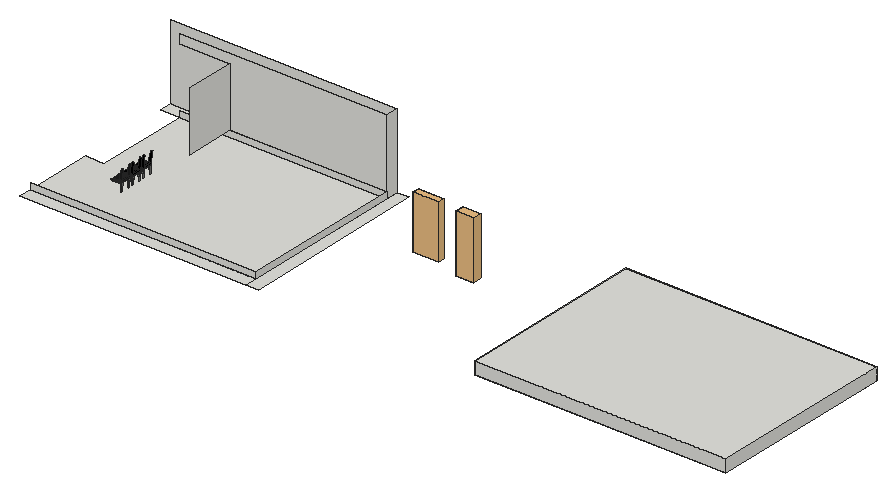
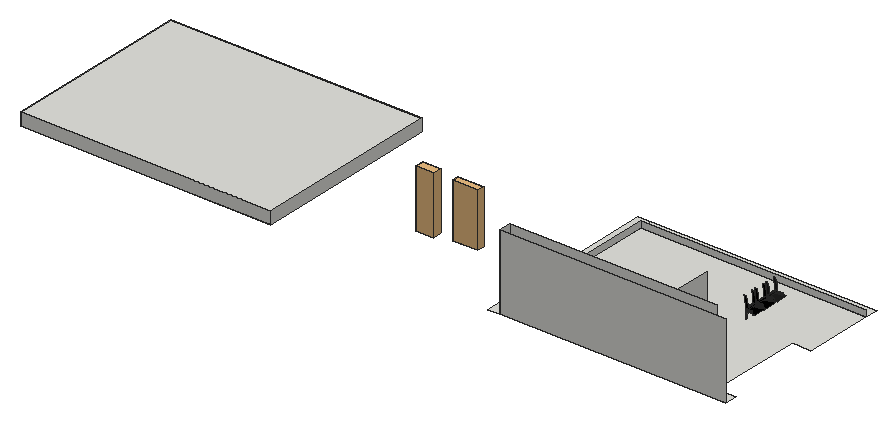
# SketchUp Ruby script. Lengths in inches.
U = 1.inch
M = Sketchup.active_model
def pt(a) = Geom::Point3d.new(a.map { |v| v * U })
def face(e, loops, mat)
  f = e.add_face(loops[0].map { |a| pt(a) })
  loops[1..].each { |l| e.add_face(l.map { |a| pt(a) }).erase! }
  f.material = f.back_material = mat if mat
  f
end
# faces: each face lists its corners as indices into pts; further lists are holes
def faces(e, pts, list, mat = nil) = list.each { |f| face(e, (f[0].is_a?(Array) ? f : [f]).map { |l| l.map { |i| pts[i] } }, mat) }
# xy, xz, yz: faces in a plane at the given z, y or x. An outline is a flat list of corners, or four numbers for a rectangle; further outlines are holes
def ring(l) = l.size == 4 ? [[l[0], l[1]], [l[2], l[1]], [l[2], l[3]], [l[0], l[3]]] : l.each_slice(2).to_a
def flat(e, list, mat, &to3) = list.each { |f| face(e, (f[0].is_a?(Array) ? f : [f]).map { |l| ring(l).map { |u, v| to3.(u, v) } }, mat) }
def xy(e, z, list, mat = nil) = flat(e, list, mat) { |x, y| [x, y, z] }
def xz(e, y, list, mat = nil) = flat(e, list, mat) { |x, z| [x, y, z] }
def yz(e, x, list, mat = nil) = flat(e, list, mat) { |y, z| [x, y, z] }
def lines(e, pts, list) = list.each { |a, b| e.add_line(pt(pts[a]), pt(pts[b])) }
# prism: a flat outline (further loops are holes) pulled along v
def prism(e, loops, v, mat = nil)
  f = face(e, loops, mat); d = Geom::Vector3d.new(v.map { |x| x * U })
  f.pushpull(f.normal.samedirection?(d) ? d.length : -d.length)
end
def box(e, o, s, mat = nil) = prism(e, [[o, [o[0] + s[0], o[1], o[2]], [o[0] + s[0], o[1] + s[1], o[2]], [o[0], o[1] + s[1], o[2]]]], [0, 0, s[2]], mat)
def at(x, y, z, deg = 0) = Geom::Transformation.translation(pt([x, y, z])) * Geom::Transformation.rotation(ORIGIN, Z_AXIS, deg.degrees)
def axes(o, x, y, z) = Geom::Transformation.new([*x, 0, *y, 0, *z, 0, *pt(o).to_a, 1])
def part(name) = M.definitions.add(name)
# library, detail: a bought-in or finely detailed component or shape, given as its bounding box
def library(name, o, s) = part(name).tap { |d| box(d.entities, o, s) }
def detail(e, o, s) = box(e.add_group.entities, o, s)
def put(e, d, t, mat = nil) = e.add_instance(d, t).tap { |i| i.material = mat if mat }
def group(e, t, mat = nil) = e.add_group.tap { |g| g.transformation = t; g.material = mat if mat }.entities
root = M.entities
M.materials.add("Color_008").color = [30, 30, 30]
M.materials.add("[Color M08]").color = [30, 30, 30]
M.materials.add("[Color M09]").color = [0, 0, 0]
M.materials.add("[Metal Seamed]").color = [118, 119, 115]
c1 = library("Group\#2",[0,0,0],[48.53,12.58,103.73])
c2 = library("Group\#1",[0,0,0],[34.5,17.48,110.79])
box(root,[894.9375,0,0],[480,360,24])
xy(root,0,[[24,0,456,24],[456,0,480,360],[24,24,24,156,60,156,60,336,456,336,456,24],[24,336,456,360]])
xy(root,12,[[146.137,88.857,146.954,89.674],[146.137,105.091,146.954,105.908],[146.137,114.763,146.954,115.58],[146.137,130.997,146.954,131.814],[146.137,140.669,146.954,141.485],
  [146.137,156.903,146.954,157.72]],"Color_008")
xy(root,26.704,[[145.473,88.193,147.618,90.338],[145.473,104.427,147.618,106.572],[145.473,114.098,147.618,116.244],[145.473,130.333,147.618,132.478],[145.473,140.004,147.618,142.15],
  [145.473,156.239,147.618,158.384]],"Color_008")
xy(root,26.704,[[132.315,87.045,130.608,87.058,128.902,87.101,127.197,87.171,129.342,87.171,129.342,89.317,127.197,89.317,127.197,105.448,129.342,105.448,129.342,107.593,127.197,107.593,128.902,107.664,130.608,107.706,132.315,107.72,134.022,107.706,135.728,107.663,137.433,107.592,139.137,107.493,140.839,107.365,142.538,107.209,144.235,107.025,145.929,106.8125,147.618,106.572,145.473,106.572,145.473,104.427,147.618,104.427,147.618,90.338,145.473,90.338,145.473,88.193,147.618,88.193,145.929,87.952,144.235,87.74,142.538,87.556,140.839,87.4,139.137,87.272,137.433,87.173,135.728,87.102,134.022,87.059]],"[Color M08]")
xy(root,26.704,[[132.315,112.95,130.608,112.964,128.902,113.007,127.197,113.077,129.342,113.077,129.342,115.223,127.197,115.223,127.197,131.354,129.342,131.354,129.342,133.499,127.197,133.499,128.902,133.57,130.608,133.612,132.315,133.626,134.022,133.612,135.728,133.569,137.433,133.498,139.137,133.398,140.839,133.271,142.538,133.115,144.235,132.931,145.929,132.718,147.618,132.478,145.473,132.478,145.473,130.333,147.618,130.333,147.618,116.244,145.473,116.244,145.473,114.098,147.618,114.098,145.929,113.858,144.235,113.646,142.538,113.462,140.839,113.306,139.137,113.178,137.433,113.079,135.728,113.008,134.022,112.965],[132.315,138.856,130.608,138.87,128.902,138.913,127.197,138.983,129.342,138.983,129.342,141.129,127.197,141.129,127.197,157.26,129.342,157.26,129.342,159.405,127.197,159.405,128.902,159.476,130.608,159.518,132.315,159.532,134.022,159.517,135.728,159.475,137.433,159.404,139.137,159.304,140.839,159.177,142.538,159.021,144.235,158.837,145.929,158.624,147.618,158.384,145.473,158.384,145.473,156.239,147.618,156.239,147.618,142.15,145.473,142.15,145.473,140.004,147.618,140.004,145.929,139.764,144.235,139.552,142.538,139.367,140.839,139.212,139.137,139.084,137.433,138.984,135.728,138.913,134.022,138.871]],"[Color M09]")
xy(root,28.845,[[144.082,88.193,147.618,106.572]],"[Color M08]")
xy(root,28.845,[[144.082,114.098,147.618,132.478],[144.082,140.004,147.618,158.384]],"[Color M09]")
xz(root,24,[[24,0,456,12]])
xz(root,88.193,[[144.082,28.845,143.95,30.816,143.898,32.79,143.926,34.764,144.034,36.736,144.222,38.701,144.488,40.658,144.834,42.602,145.258,44.53,145.759,46.44,146.337,48.328,146.991,50.191,147.719,52.027,150.17,52.027,149.772,50.121,149.407,48.208,149.076,46.29,148.779,44.365,148.515,42.436,148.285,40.503,148.089,38.566,147.927,36.626,147.799,34.683,147.705,32.738,147.645,30.792,147.618,28.845]],"[Color M08]")
xz(root,106.572,[[144.082,28.845,147.618,28.845,147.645,30.792,147.705,32.738,147.799,34.683,147.927,36.626,148.089,38.566,148.285,40.503,148.515,42.436,148.779,44.365,149.076,46.29,149.407,48.208,149.772,50.121,150.17,52.027,147.719,52.027,146.991,50.191,146.337,48.328,145.759,46.44,145.258,44.53,144.834,42.602,144.488,40.658,144.222,38.701,144.034,36.736,143.926,34.764,143.898,32.79,143.95,30.816]],"[Color M08]")
xz(root,114.098,[[144.082,28.845,143.95,30.816,143.898,32.79,143.926,34.764,144.034,36.736,144.222,38.701,144.488,40.658,144.834,42.602,145.258,44.53,145.759,46.44,146.337,48.328,146.991,50.191,147.719,52.027,150.17,52.027,149.772,50.121,149.407,48.208,149.076,46.29,148.779,44.365,148.515,42.436,148.285,40.503,148.089,38.566,147.927,36.626,147.799,34.683,147.705,32.738,147.645,30.792,147.618,28.845]],"[Color M09]")
xz(root,132.478,[[144.082,28.845,147.618,28.845,147.645,30.792,147.705,32.738,147.799,34.683,147.927,36.626,148.089,38.566,148.285,40.503,148.515,42.436,148.779,44.365,149.076,46.29,149.407,48.208,149.772,50.121,150.17,52.027,147.719,52.027,146.991,50.191,146.337,48.328,145.759,46.44,145.258,44.53,144.834,42.602,144.488,40.658,144.222,38.701,144.034,36.736,143.926,34.764,143.898,32.79,143.95,30.816]],"[Color M09]")
xz(root,140.004,[[144.082,28.845,143.95,30.816,143.898,32.79,143.926,34.764,144.034,36.736,144.222,38.701,144.488,40.658,144.834,42.602,145.258,44.53,145.759,46.44,146.337,48.328,146.991,50.191,147.719,52.027,150.17,52.027,149.772,50.121,149.407,48.208,149.076,46.29,148.779,44.365,148.515,42.436,148.285,40.503,148.089,38.566,147.927,36.626,147.799,34.683,147.705,32.738,147.645,30.792,147.618,28.845]],"[Color M09]")
xz(root,158.384,[[144.082,28.845,147.618,28.845,147.645,30.792,147.705,32.738,147.799,34.683,147.927,36.626,148.089,38.566,148.285,40.503,148.515,42.436,148.779,44.365,149.076,46.29,149.407,48.208,149.772,50.121,150.17,52.027,147.719,52.027,146.991,50.191,146.337,48.328,145.759,46.44,145.258,44.53,144.834,42.602,144.488,40.658,144.222,38.701,144.034,36.736,143.926,34.764,143.898,32.79,143.95,30.816]],"[Color M09]")
xz(root,336,[[60,0,456,12],[156,12,456,12,456,144,60,144,60,126,156,126]])
xz(root,360,[[24,0,456,144]])
yz(root,147.618,[[88.193,26.704,106.572,28.845]],"[Color M08]")
yz(root,147.618,[[114.098,26.704,132.478,28.845],[140.004,26.704,158.384,28.845]],"[Color M09]")
yz(root,156,[[240,12,336,126]])
yz(root,456,[[24,0,336,12],[336,0,360,144]])
p = [[145.473,90.338,26.704],[146.137,89.674,12],[146.137,88.857,12],[145.473,88.193,26.704],[146.954,88.857,12],[147.618,88.193,26.704],
  [146.954,89.674,12],[147.618,90.338,26.704],[146.137,105.091,12],[145.473,104.427,26.704],[145.473,106.572,26.704],[146.137,105.908,12],
  [146.954,105.091,12],[147.618,104.427,26.704],[146.954,105.908,12],[147.618,106.572,26.704],[145.473,116.244,26.704],[146.137,115.58,12],
  [146.137,114.763,12],[145.473,114.098,26.704],[146.954,114.763,12],[147.618,114.098,26.704],[146.954,115.58,12],[147.618,116.244,26.704],
  [146.137,130.997,12],[145.473,130.333,26.704],[145.473,132.478,26.704],[146.137,131.814,12],[146.954,130.997,12],[147.618,130.333,26.704],
  [146.954,131.814,12],[147.618,132.478,26.704],[145.473,142.15,26.704],[146.137,141.485,12],[146.137,140.669,12],[145.473,140.004,26.704],
  [146.954,140.669,12],[147.618,140.004,26.704],[146.954,141.485,12],[147.618,142.15,26.704],[146.137,156.903,12],[145.473,156.239,26.704],
  [145.473,158.384,26.704],[146.137,157.72,12],[146.954,156.903,12],[147.618,156.239,26.704],[146.954,157.72,12],[147.618,158.384,26.704],
  [135.728,87.102,28.845],[135.728,87.102,26.704],[134.022,87.059,26.704],[134.022,87.059,28.845],[137.433,87.173,26.704],[137.433,87.173,28.845],
  [139.137,87.272,26.704],[139.137,87.272,28.845],[140.839,87.4,26.704],[140.839,87.4,28.845],[142.538,87.556,26.704],[142.538,87.556,28.845],
  [144.235,87.74,26.704],[144.235,87.74,28.845],[145.929,87.952,26.704],[145.929,87.952,28.845],[147.618,88.193,28.845],[145.929,106.8125,26.704],
  [145.929,106.8125,28.845],[147.618,106.572,28.845],[144.235,107.025,26.704],[144.235,107.025,28.845],[142.538,107.209,26.704],[142.538,107.209,28.845],
  [140.839,107.365,26.704],[140.839,107.365,28.845],[139.137,107.493,26.704],[139.137,107.493,28.845],[137.433,107.592,26.704],[137.433,107.592,28.845],
  [135.728,107.663,26.704],[135.728,107.663,28.845],[134.022,107.706,28.845],[134.022,107.706,26.704],[135.728,113.008,28.845],[135.728,113.008,26.704],
  [134.022,112.965,26.704],[134.022,112.965,28.845],[137.433,113.079,26.704],[137.433,113.079,28.845],[139.137,113.178,26.704],[139.137,113.178,28.845],
  [140.839,113.306,26.704],[140.839,113.306,28.845],[142.538,113.462,26.704],[142.538,113.462,28.845],[144.235,113.646,26.704],[144.235,113.646,28.845],
  [145.929,113.858,26.704],[145.929,113.858,28.845],[147.618,114.098,28.845],[145.929,132.718,26.704],[145.929,132.718,28.845],[147.618,132.478,28.845],
  [144.235,132.931,26.704],[144.235,132.931,28.845],[142.538,133.115,26.704],[142.538,133.115,28.845],[140.839,133.271,26.704],[140.839,133.271,28.845],
  [139.137,133.398,26.704],[139.137,133.398,28.845],[137.433,133.498,26.704],[137.433,133.498,28.845],[135.728,133.569,26.704],[135.728,133.569,28.845],
  [134.022,133.612,28.845],[134.022,133.612,26.704],[135.728,138.913,28.845],[135.728,138.913,26.704],[134.022,138.871,26.704],[134.022,138.871,28.845],
  [137.433,138.984,26.704],[137.433,138.984,28.845],[139.137,139.084,26.704],[139.137,139.084,28.845],[140.839,139.212,26.704],[140.839,139.212,28.845],
  [142.538,139.367,26.704],[142.538,139.367,28.845],[144.235,139.552,26.704],[144.235,139.552,28.845],[145.929,139.764,26.704],[145.929,139.764,28.845],
  [147.618,140.004,28.845],[145.929,158.624,26.704],[145.929,158.624,28.845],[147.618,158.384,28.845],[144.235,158.837,26.704],[144.235,158.837,28.845],
  [142.538,159.021,26.704],[142.538,159.021,28.845],[140.839,159.177,26.704],[140.839,159.177,28.845],[139.137,159.304,26.704],[139.137,159.304,28.845],
  [137.433,159.404,26.704],[137.433,159.404,28.845],[135.728,159.475,26.704],[135.728,159.475,28.845],[134.022,159.517,28.845],[134.022,159.517,26.704],
  [135.728,87.111,28.992],[134.021,87.069,28.992],[137.433,87.182,28.992],[139.136,87.282,28.992],[140.838,87.409,28.992],[142.538,87.565,28.992],
  [144.234,87.749,28.992],[145.927,87.962,28.992],[147.609,88.201,28.992],[143.95,88.193,30.816],[144.082,88.193,28.845],[144.082,106.572,28.845],
  [143.95,106.572,30.816],[147.609,106.564,28.992],[147.645,88.193,30.792],[147.645,106.572,30.792],[145.927,106.803,28.992],[144.234,107.015,28.992],
  [142.538,107.199,28.992],[140.838,107.355,28.992],[139.136,107.483,28.992],[137.433,107.582,28.992],[135.728,107.653,28.992],[134.021,107.696,28.992],
  [135.728,113.017,28.992],[134.021,112.974,28.992],[137.433,113.088,28.992],[139.136,113.1875,28.992],[140.838,113.315,28.992],[142.538,113.471,28.992],
  [144.234,113.655,28.992],[145.927,113.868,28.992],[147.609,114.107,28.992],[143.95,114.098,30.816],[144.082,114.098,28.845],[144.082,132.478,28.845],
  [143.95,132.478,30.816],[147.609,132.47,28.992],[147.645,114.098,30.792],[147.645,132.478,30.792],[145.927,132.709,28.992],[144.234,132.921,28.992],
  [142.538,133.105,28.992],[140.838,133.261,28.992],[139.136,133.389,28.992],[137.433,133.488,28.992],[135.728,133.559,28.992],[134.021,133.602,28.992],
  [135.728,138.923,28.992],[134.021,138.88,28.992],[137.433,138.994,28.992],[139.136,139.093,28.992],[140.838,139.221,28.992],[142.538,139.377,28.992],
  [144.234,139.561,28.992],[145.927,139.773,28.992],[147.609,140.013,28.992],[143.95,140.004,30.816],[144.082,140.004,28.845],[144.082,158.384,28.845],
  [143.95,158.384,30.816],[147.609,158.376,28.992],[147.645,140.004,30.792],[147.645,158.384,30.792],[145.927,158.615,28.992],[144.234,158.827,28.992],
  [142.538,159.011,28.992],[140.838,159.167,28.992],[139.136,159.295,28.992],[137.433,159.394,28.992],[135.728,159.465,28.992],[134.021,159.508,28.992],
  [135.726,87.14,29.137],[134.021,87.097,29.137],[137.431,87.211,29.137],[139.134,87.31,29.137],[140.836,87.438,29.137],[142.535,87.594,29.137],
  [144.231,87.778,29.137],[145.924,87.99,29.137],[147.58,88.226,29.137],[147.58,106.539,29.137],[147.58,97.382,29.137],[145.924,106.774,29.137],
  [144.231,106.987,29.137],[142.535,107.171,29.137],[140.836,107.327,29.137],[139.134,107.454,29.137],[137.431,107.554,29.137],[135.727,107.625,29.137],
  [134.021,107.667,29.137],[135.726,113.046,29.137],[134.021,113.003,29.137],[137.431,113.117,29.137],[139.134,113.216,29.137],[140.836,113.344,29.137],
  [142.535,113.5,29.137],[144.231,113.684,29.137],[145.924,113.896,29.137],[147.58,114.132,29.137],[147.58,132.445,29.137],[147.58,123.288,29.137],
  [145.924,132.68,29.137],[144.231,132.893,29.137],[142.535,133.077,29.137],[140.836,133.233,29.137],[139.134,133.36,29.137],[137.431,133.46,29.137],
  [135.727,133.531,29.137],[134.021,133.573,29.137],[135.726,138.952,29.137],[134.021,138.909,29.137],[137.431,139.023,29.137],[139.134,139.122,29.137],
  [140.836,139.25,29.137],[142.535,139.406,29.137],[144.231,139.59,29.137],[145.924,139.802,29.137],[147.58,140.038,29.137],[147.58,158.351,29.137],
  [147.58,149.194,29.137],[145.924,158.586,29.137],[144.231,158.798,29.137],[142.535,158.983,29.137],[140.836,159.138,29.137],[139.134,159.266,29.137],
  [137.431,159.365,29.137],[135.727,159.436,29.137],[134.021,159.479,29.137],[134.02,87.145,29.276],[135.724,87.187,29.276],[137.429,87.258,29.276],
  [135.726,87.187,29.276],[139.131,87.358,29.276],[140.832,87.485,29.276],[142.53,87.641,29.276],[144.225,87.825,29.276],[145.917,88.037,29.276],
  [147.533,88.267,29.276],[147.533,97.382,29.276],[147.533,106.498,29.276],[145.917,106.728,29.276],[144.225,106.94,29.276],[142.53,107.124,29.276],
  [140.832,107.279,29.276],[139.131,107.407,29.276],[137.429,107.506,29.276],[135.724,107.577,29.276],[135.726,107.577,29.276],[134.02,107.62,29.276],
  [134.02,113.05,29.276],[135.724,113.093,29.276],[137.429,113.164,29.276],[135.726,113.093,29.276],[139.131,113.263,29.276],[140.832,113.391,29.276],
  [142.53,113.547,29.276],[144.225,113.731,29.276],[145.917,113.943,29.276],[147.533,114.173,29.276],[147.533,123.288,29.276],[147.533,132.404,29.276],
  [145.917,132.633,29.276],[144.225,132.846,29.276],[142.53,133.03,29.276],[140.832,133.185,29.276],[139.131,133.313,29.276],[137.429,133.412,29.276],
  [135.724,133.483,29.276],[135.726,133.483,29.276],[134.02,133.526,29.276],[134.02,138.956,29.276],[135.724,138.999,29.276],[137.429,139.07,29.276],
  [135.726,138.999,29.276],[139.131,139.169,29.276],[140.832,139.297,29.276],[142.53,139.453,29.276],[144.225,139.637,29.276],[145.917,139.849,29.276],
  [147.533,140.079,29.276],[147.533,149.194,29.276],[147.533,158.31,29.276],[145.917,158.539,29.276],[144.225,158.751,29.276],[142.53,158.935,29.276],
  [140.832,159.091,29.276],[139.131,159.219,29.276],[137.429,159.318,29.276],[135.724,159.389,29.276],[135.726,159.389,29.276],[134.02,159.432,29.276],
  [134.019,87.21,29.408],[135.722,87.252,29.408],[135.724,87.252,29.408],[137.426,87.323,29.408],[139.127,87.423,29.408],[140.826,87.55,29.408],
  [142.523,87.706,29.408],[144.218,87.89,29.408],[145.909,88.102,29.408],[147.468,88.323,29.408],[147.468,97.382,29.408],[147.468,106.441,29.408],
  [145.909,106.663,29.408],[144.218,106.875,29.408],[142.523,107.059,29.408],[140.826,107.215,29.408],[139.127,107.342,29.408],[137.426,107.441,29.408],
  [135.724,107.512,29.408],[135.722,107.512,29.408],[134.019,107.555,29.408],[134.019,113.116,29.408],[135.722,113.158,29.408],[135.724,113.158,29.408],
  [137.426,113.229,29.408],[139.127,113.328,29.408],[140.826,113.456,29.408],[142.523,113.612,29.408],[144.218,113.795,29.408],[145.909,114.007,29.408],
  [147.468,114.229,29.408],[147.468,123.288,29.408],[147.468,132.347,29.408],[145.909,132.569,29.408],[144.218,132.781,29.408],[142.523,132.965,29.408],
  [140.826,133.121,29.408],[139.127,133.248,29.408],[137.426,133.347,29.408],[135.724,133.418,29.408],[135.722,133.418,29.408],[134.019,133.461,29.408],
  [134.019,139.021,29.408],[135.722,139.064,29.408],[135.724,139.064,29.408],[137.426,139.135,29.408],[139.127,139.234,29.408],[140.826,139.362,29.408],
  [142.523,139.517,29.408],[144.218,139.701,29.408],[145.909,139.913,29.408],[147.468,140.135,29.408],[147.468,149.194,29.408],[147.468,158.253,29.408],
  [145.909,158.475,29.408],[144.218,158.687,29.408],[142.523,158.871,29.408],[140.826,159.026,29.408],[139.127,159.154,29.408],[137.426,159.253,29.408],
  [135.722,159.324,29.408],[134.019,159.367,29.408],[135.724,159.324,29.408],[134.018,87.291,29.531],[135.718,87.334,29.531],[135.722,87.334,29.531],
  [137.421,87.405,29.531],[139.121,87.504,29.531],[140.82,87.631,29.531],[142.515,87.787,29.531],[144.208,87.971,29.531],[145.898,88.183,29.531],
  [147.386,88.394,29.531],[147.386,97.382,29.531],[147.386,106.37,29.531],[145.898,106.582,29.531],[144.208,106.794,29.531],[142.515,106.978,29.531],
  [140.82,107.133,29.531],[139.121,107.261,29.531],[137.421,107.36,29.531],[135.718,107.431,29.531],[134.018,107.473,29.531],[135.722,107.431,29.531],
  [134.018,113.197,29.531],[135.718,113.24,29.531],[135.722,113.24,29.531],[137.421,113.311,29.531],[139.121,113.41,29.531],[140.82,113.537,29.531],
  [142.515,113.693,29.531],[144.208,113.877,29.531],[145.898,114.088,29.531],[147.386,114.3,29.531],[147.386,123.288,29.531],[147.386,132.276,29.531],
  [145.898,132.488,29.531],[144.208,132.7,29.531],[142.515,132.883,29.531],[140.82,133.039,29.531],[139.121,133.166,29.531],[137.421,133.266,29.531],
  [135.718,133.337,29.531],[134.018,133.379,29.531],[135.722,133.336,29.531],[134.018,139.103,29.531],[135.718,139.146,29.531],[135.722,139.146,29.531],
  [137.421,139.217,29.531],[139.121,139.316,29.531],[140.82,139.443,29.531],[142.515,139.599,29.531],[144.208,139.783,29.531],[145.898,139.994,29.531],
  [147.386,140.206,29.531],[147.386,149.194,29.531],[147.386,158.182,29.531],[145.898,158.394,29.531],[144.208,158.606,29.531],[142.515,158.789,29.531],
  [140.82,158.945,29.531],[139.121,159.072,29.531],[137.421,159.171,29.531],[135.718,159.242,29.531],[134.018,159.285,29.531],[135.722,159.242,29.531],
  [135.72,87.431,29.641],[135.714,87.431,29.641],[137.417,87.502,29.641],[139.115,87.601,29.641],[140.811,87.728,29.641],[142.506,87.884,29.641],
  [144.197,88.067,29.641],[145.885,88.279,29.641],[147.289,88.479,29.641],[147.289,97.382,29.641],[147.289,106.286,29.641],[145.885,106.486,29.641],
  [144.197,106.697,29.641],[142.506,106.881,29.641],[140.811,107.036,29.641],[139.115,107.164,29.641],[137.417,107.263,29.641],[135.72,107.333,29.641],
  [135.714,107.334,29.641],[134.016,139.2,29.641],[135.714,139.243,29.641],[135.72,139.243,29.641],[137.417,139.314,29.641],[139.115,139.413,29.641],
  [140.811,139.54,29.641],[142.506,139.695,29.641],[144.197,139.879,29.641],[145.885,140.091,29.641],[147.289,140.29,29.641],[147.289,149.194,29.641],
  [147.289,158.098,29.641],[145.885,158.298,29.641],[144.197,158.509,29.641],[142.506,158.693,29.641],[140.811,158.848,29.641],[139.115,158.975,29.641],
  [137.417,159.075,29.641],[135.72,159.145,29.641],[135.714,159.145,29.641]]
faces(root,p,[[0,1,2,3],[3,2,4,5],[6,7,5,4],[1,0,7,6],[8,9,10,11],[9,8,12,13],[13,12,14,15],[11,10,15,14],
  [16,17,18,19],[19,18,20,21],[22,23,21,20],[17,16,23,22],[24,25,26,27],[25,24,28,29],[29,28,30,31],[27,26,31,30],
  [32,33,34,35],[35,34,36,37],[38,39,37,36],[33,32,39,38],[40,41,42,43],[41,40,44,45],[45,44,46,47],[43,42,47,46]],"[Metal Seamed]")
faces(root,p,[[48,49,50,51],[48,49,52,53],[53,52,54,55],[55,54,56,57],[57,56,58,59],[59,58,60,61],[61,60,62,63],[63,62,5,64],
  [65,66,67,15],[68,69,66,65],[70,71,69,68],[72,73,71,70],[74,75,73,72],[76,77,75,74],[78,79,77,76],[78,79,80,81],
  [150,48,51,151],[150,48,53,152],[152,53,55,153],[153,55,57,154],[154,57,59,155],[155,59,61,156],[156,61,63,157],[157,63,64,158],
  [159,160,161,162],[158,64,67,163],[64,164,165,67],[66,166,163,67],[69,167,166,66],[71,168,167,69],[73,169,168,71],[75,170,169,73],
  [77,171,170,75],[79,172,171,77],[79,172,173,80],[222,150,151,223],[150,152,224,222],[224,152,153,225],[225,153,154,226],[226,154,155,227],
  [227,155,156,228],[228,156,157,229],[229,157,158,230],[230,158,163,231,232],[166,233,231,163],[167,234,233,166],[168,235,234,167],[169,236,235,168],
  [170,237,236,169],[171,238,237,170],[172,239,240,173],[171,172,239,238],[222,223,279,280],[280,222,224,281,282],[281,224,225,283],[283,225,226,284],
  [284,226,227,285],[285,227,228,286],[286,228,229,287],[287,229,230,288],[288,230,232,289],[231,290,289,232],[233,291,290,231],[234,292,291,233],
  [235,293,292,234],[236,294,293,235],[237,295,294,236],[238,296,295,237],[239,297,298,296,238],[240,239,297,299],[280,279,342,343],[344,343,280,282],
  [282,281,345,344],[345,281,283,346],[346,283,284,347],[347,284,285,348],[348,285,286,349],[349,286,287,350],[350,287,288,351],[351,288,289,352],
  [290,353,352,289],[291,354,353,290],[292,355,354,291],[293,356,355,292],[294,357,356,293],[295,358,357,294],[296,359,358,295],[296,298,360,359],
  [299,297,361,362],[360,361,297,298],[343,342,405,406],[406,407,344,343],[344,345,408,407],[408,345,346,409],[409,346,347,410],[410,347,348,411],
  [411,348,349,412],[412,349,350,413],[413,350,351,414],[414,351,352,415],[353,416,415,352],[354,417,416,353],[355,418,417,354],[356,419,418,355],
  [357,420,419,356],[358,421,420,357],[359,422,421,358],[362,361,423,424],[423,425,360,361],[359,360,425,422],[468,469,406,407],[407,408,470,468],
  [470,408,409,471],[471,409,410,472],[472,410,411,473],[473,411,412,474],[474,412,413,475],[475,413,414,476],[476,414,415,477],[416,478,477,415],
  [417,479,478,416],[418,480,479,417],[419,481,480,418],[420,482,481,419],[421,483,482,420],[422,484,483,421],[485,486,423,425],[422,425,485,484]],"[Color M08]")
faces(root,p,[[82,83,84,85],[82,83,86,87],[87,86,88,89],[89,88,90,91],[91,90,92,93],[93,92,94,95],[95,94,96,97],[97,96,21,98],
  [99,100,101,31],[102,103,100,99],[104,105,103,102],[106,107,105,104],[108,109,107,106],[110,111,109,108],[112,113,111,110],[112,113,114,115],
  [116,117,118,119],[116,117,120,121],[121,120,122,123],[123,122,124,125],[125,124,126,127],[127,126,128,129],[129,128,130,131],[131,130,37,132],
  [133,134,135,47],[136,137,134,133],[138,139,137,136],[140,141,139,138],[142,143,141,140],[144,145,143,142],[146,147,145,144],[146,147,148,149],
  [174,82,85,175],[174,82,87,176],[176,87,89,177],[177,89,91,178],[178,91,93,179],[179,93,95,180],[180,95,97,181],[181,97,98,182],
  [183,184,185,186],[182,98,101,187],[98,188,189,101],[100,190,187,101],[103,191,190,100],[105,192,191,103],[107,193,192,105],[109,194,193,107],
  [111,195,194,109],[113,196,195,111],[113,196,197,114],[198,116,119,199],[198,116,121,200],[200,121,123,201],[201,123,125,202],[202,125,127,203],
  [203,127,129,204],[204,129,131,205],[205,131,132,206],[207,208,209,210],[206,132,135,211],[132,212,213,135],[134,214,211,135],[137,215,214,134],
  [139,216,215,137],[141,217,216,139],[143,218,217,141],[145,219,218,143],[147,220,219,145],[147,220,221,148],[241,174,175,242],[174,176,243,241],
  [243,176,177,244],[244,177,178,245],[245,178,179,246],[246,179,180,247],[247,180,181,248],[248,181,182,249],[249,182,187,250,251],[190,252,250,187],
  [191,253,252,190],[192,254,253,191],[193,255,254,192],[194,256,255,193],[195,257,256,194],[196,258,259,197],[195,196,258,257],[260,198,199,261],
  [198,200,262,260],[262,200,201,263],[263,201,202,264],[264,202,203,265],[265,203,204,266],[266,204,205,267],[267,205,206,268],[268,206,211,269,270],
  [214,271,269,211],[215,272,271,214],[216,273,272,215],[217,274,273,216],[218,275,274,217],[219,276,275,218],[220,277,278,221],[219,220,277,276],
  [241,242,300,301],[301,241,243,302,303],[302,243,244,304],[304,244,245,305],[305,245,246,306],[306,246,247,307],[307,247,248,308],[308,248,249,309],
  [309,249,251,310],[250,311,310,251],[252,312,311,250],[253,313,312,252],[254,314,313,253],[255,315,314,254],[256,316,315,255],[257,317,316,256],
  [258,318,319,317,257],[259,258,318,320],[260,261,321,322],[322,260,262,323,324],[323,262,263,325],[325,263,264,326],[326,264,265,327],[327,265,266,328],
  [328,266,267,329],[329,267,268,330],[330,268,270,331],[269,332,331,270],[271,333,332,269],[272,334,333,271],[273,335,334,272],[274,336,335,273],
  [275,337,336,274],[276,338,337,275],[277,339,340,338,276],[278,277,339,341],[301,300,363,364],[365,364,301,303],[303,302,366,365],[366,302,304,367],
  [367,304,305,368],[368,305,306,369],[369,306,307,370],[370,307,308,371],[371,308,309,372],[372,309,310,373],[311,374,373,310],[312,375,374,311],
  [313,376,375,312],[314,377,376,313],[315,378,377,314],[316,379,378,315],[317,380,379,316],[317,319,381,380],[320,318,382,383],[381,382,318,319],
  [322,321,384,385],[386,385,322,324],[324,323,387,386],[387,323,325,388],[388,325,326,389],[389,326,327,390],[390,327,328,391],[391,328,329,392],
  [392,329,330,393],[393,330,331,394],[332,395,394,331],[333,396,395,332],[334,397,396,333],[335,398,397,334],[336,399,398,335],[337,400,399,336],
  [338,401,400,337],[341,339,402,403],[404,402,339,340],[338,340,404,401],[364,363,426,427],[427,428,365,364],[365,366,429,428],[429,366,367,430],
  [430,367,368,431],[431,368,369,432],[432,369,370,433],[433,370,371,434],[434,371,372,435],[435,372,373,436],[374,437,436,373],[375,438,437,374],
  [376,439,438,375],[377,440,439,376],[378,441,440,377],[379,442,441,378],[380,443,442,379],[383,382,444,445],[444,446,381,382],[380,381,446,443],
  [385,384,447,448],[448,449,386,385],[386,387,450,449],[450,387,388,451],[451,388,389,452],[452,389,390,453],[453,390,391,454],[454,391,392,455],
  [455,392,393,456],[456,393,394,457],[395,458,457,394],[396,459,458,395],[397,460,459,396],[398,461,460,397],[399,462,461,398],[400,463,462,399],
  [401,464,463,400],[403,402,465,466],[465,467,404,402],[401,404,467,464],[448,447,487,488],[489,488,448,449],[449,450,490,489],[490,450,451,491],
  [491,451,452,492],[492,452,453,493],[493,453,454,494],[494,454,455,495],[495,455,456,496],[496,456,457,497],[458,498,497,457],[459,499,498,458],
  [460,500,499,459],[461,501,500,460],[462,502,501,461],[463,503,502,462],[464,504,503,463],[505,506,465,467],[464,467,505,504]],"[Color M09]")
put(root,c1,at(596.74,224.45,6.26))
put(root,c2,at(682.03,219.97,-1.8125))
